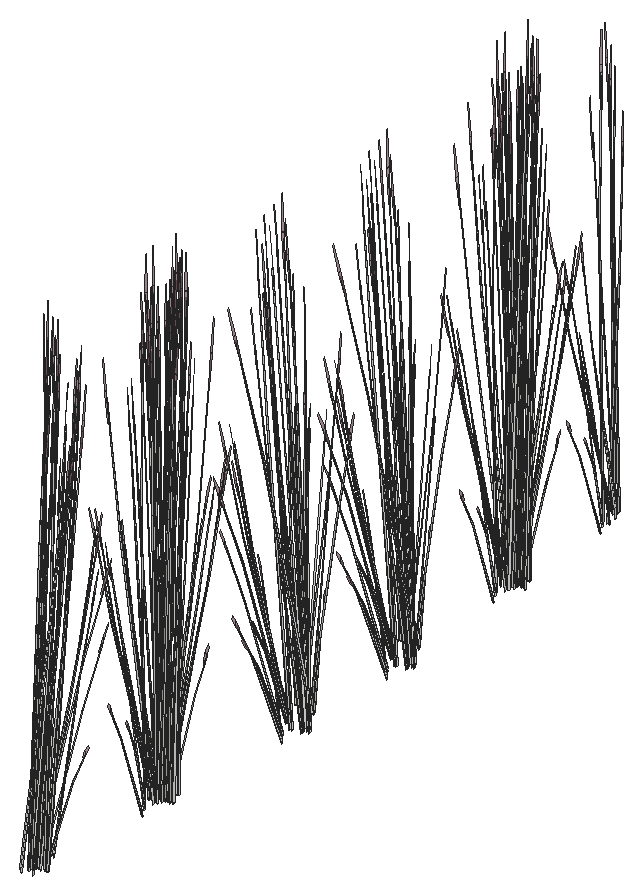
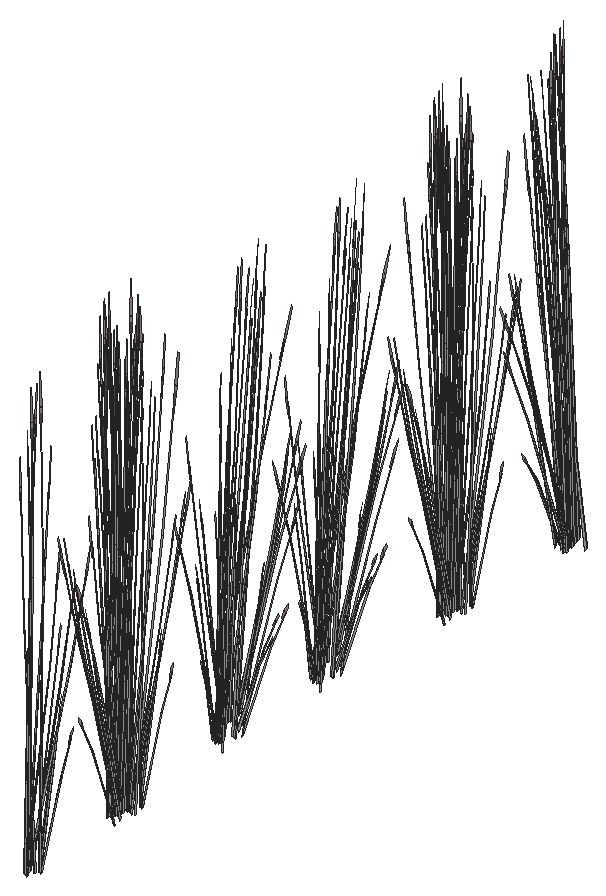
# SketchUp Ruby script. Lengths in inches.
U = 1.inch
M = Sketchup.active_model
def pt(a) = Geom::Point3d.new(a.map { |v| v * U })
def face(e, loops, mat)
  f = e.add_face(loops[0].map { |a| pt(a) })
  loops[1..].each { |l| e.add_face(l.map { |a| pt(a) }).erase! }
  f.material = f.back_material = mat if mat
  f
end
# faces: each face lists its corners as indices into pts; further lists are holes
def faces(e, pts, list, mat = nil) = list.each { |f| face(e, (f[0].is_a?(Array) ? f : [f]).map { |l| l.map { |i| pts[i] } }, mat) }
# xy, xz, yz: faces in a plane at the given z, y or x. An outline is a flat list of corners, or four numbers for a rectangle; further outlines are holes
def ring(l) = l.size == 4 ? [[l[0], l[1]], [l[2], l[1]], [l[2], l[3]], [l[0], l[3]]] : l.each_slice(2).to_a
def flat(e, list, mat, &to3) = list.each { |f| face(e, (f[0].is_a?(Array) ? f : [f]).map { |l| ring(l).map { |u, v| to3.(u, v) } }, mat) }
def xy(e, z, list, mat = nil) = flat(e, list, mat) { |x, y| [x, y, z] }
def xz(e, y, list, mat = nil) = flat(e, list, mat) { |x, z| [x, y, z] }
def yz(e, x, list, mat = nil) = flat(e, list, mat) { |y, z| [x, y, z] }
def lines(e, pts, list) = list.each { |a, b| e.add_line(pt(pts[a]), pt(pts[b])) }
# prism: a flat outline (further loops are holes) pulled along v
def prism(e, loops, v, mat = nil)
  f = face(e, loops, mat); d = Geom::Vector3d.new(v.map { |x| x * U })
  f.pushpull(f.normal.samedirection?(d) ? d.length : -d.length)
end
def box(e, o, s, mat = nil) = prism(e, [[o, [o[0] + s[0], o[1], o[2]], [o[0] + s[0], o[1] + s[1], o[2]], [o[0], o[1] + s[1], o[2]]]], [0, 0, s[2]], mat)
def at(x, y, z, deg = 0) = Geom::Transformation.translation(pt([x, y, z])) * Geom::Transformation.rotation(ORIGIN, Z_AXIS, deg.degrees)
def axes(o, x, y, z) = Geom::Transformation.new([*x, 0, *y, 0, *z, 0, *pt(o).to_a, 1])
def part(name) = M.definitions.add(name)
# library, detail: a bought-in or finely detailed component or shape, given as its bounding box
def library(name, o, s) = part(name).tap { |d| box(d.entities, o, s) }
def detail(e, o, s) = box(e.add_group.entities, o, s)
def put(e, d, t, mat = nil) = e.add_instance(d, t).tap { |i| i.material = mat if mat }
def group(e, t, mat = nil) = e.add_group.tap { |g| g.transformation = t; g.material = mat if mat }.entities
root = M.entities
M.materials.add("LightPink_Translucent").color = [144, 107, 117]
M.materials["LightPink_Translucent"].alpha = 0.75
c1 = part("blade")
p = [[2.15,0.21,22],[0,0.17,0],[0.09,0.45,0],[2.18,0.31,22],[2.29,0.31,22],[0.38,0.45,0],
  [2.48,0.24,33],[2.49,0.24,33],[2.48,0.22,33]]
faces(c1.entities,p,[[0,1,2,3],[4,5,2,3],[6,3,4,7],[8,0,3,6]])
c2 = part("seeds")
p = [[0.3,-0.1,1.38],[-0.01,-0.03,1.59],[-0.01,-0.03,0.03],[0.14,-0.07,-0.07],[0.29,-0.03,3],[0.15,0.01,3.11]]
faces(c2.entities,p,[[0,1,2,3],[1,0,4,5]],"LightPink_Translucent")
c3 = part("blade with seeds")
put(c3.entities,c1,at(0,0,0))
put(c3.entities,c2,axes([2.4,0.25,30.99],[1.5799,-0.05474,1.17369],[-0.12525,1.92788,0.29478],[-0.07173,-0.02425,1.56792]))
put(root,c3,axes([397.25,199,1.59],[-0.3474,0.18671,1.28929],[-0.11057,-0.53572,0.50096],[0.21332,0.00891,1.46642]))
put(root,c3,axes([398.18,199.14,2.62],[0.06809,-0.4162,0.1448],[0.33266,0.07225,-0.41347],[0.06054,0.04274,1.26744]))
put(root,c3,axes([398.04,199.25,2.72],[-0.21202,-0.39143,0.44739],[0.32115,-0.27564,-0.21531],[0.06861,0.04843,1.43643]))
put(root,c3,axes([398.15,199.27,2.67],[0.35635,-0.30962,-0.29095],[0.23697,0.43749,-0.50002],[0.08792,0.04443,1.59708]))
put(root,c3,axes([398.42,199.78,2.21],[0.39487,0,0],[0,0.48281,0],[0,0,1.78407]))
put(root,c3,axes([398.53,198.65,2.47],[-0.37926,0.12378,0.17642],[-0.09365,-0.46065,0.35086],[0.03382,0.06712,1.60407]))
put(root,c3,axes([398.95,198.625,2.03],[0.08291,0.40636,-0.30978],[-0.32928,0.11539,0.30978],[0.06638,0.04686,1.38974]))
put(root,c3,axes([398.29,199.53,2.38],[-0.44609,-0.09826,0.49198],[0.09078,-0.55493,0.19306],[0.06519,0.05359,1.70813]))
put(root,c3,axes([398.37,200.85,2.18],[0.37054,-0.15823,-0.19198],[0.1302,0.45581,0.00008],[0.0409,-0.01749,1.73897]))
put(root,c3,axes([398.41,199.99,2.21],[0.24637,0.30123,0],[-0.24637,0.30123,0],[0,0,1.69266]))
put(root,c3,axes([398.41,199.63,2.72],[0.17124,-0.42022,0.44739],[0.35581,0.20224,-0.21531],[0,0.09687,1.43643]))
put(root,c3,axes([398.34,199.875,2.29],[0,0.53934,-0.05637],[-0.44133,0,0],[0,0.01695,1.79368]))
put(root,c3,axes([398.37,199.49,2.21],[0.21202,0.39143,-0.44739],[-0.32115,0.27564,0.21531],[0.06861,0.04843,1.43643]))
put(root,c3,axes([399.3,199.87,2.48],[0,-0.46636,0.49651],[0.39487,0,0],[0,0.10622,1.57504]))
put(root,c3,axes([398.55,199.73,2.62],[0.32884,-0.136,0.1448],[0.11516,0.38837,-0.41347],[0,0.08547,1.26744]))
put(root,c3,axes([398.26,201.09,2.2],[0.35581,0.20937,0],[-0.17124,0.43505,0],[0,0,1.74954]))
put(root,c3,axes([398.13,200.92,2.29],[0.15345,0.53576,-0.06012],[-0.43845,0.18773,0],[0.00536,0.01871,1.72173]))
put(root,c3,axes([399.57,199.95,2.375],[0.44133,0,0],[0,0.52122,-0.51607],[0,0.11871,1.63711]))
put(root,c3,axes([399.4,200.22,2.2],[-0.44111,-0.00373,-0.04976],[0,-0.52122,0.49943],[-0.01386,0.11865,1.58352]))
put(root,c3,axes([398.44,199.76,2.67],[0.39748,0.22252,-0.29095],[-0.19139,0.46966,-0.50002],[0.01249,0.11531,1.59708]))
put(root,c3,axes([399.3,200.29,2.03],[-0.24637,0.29097,-0.30978],[-0.24637,-0.29097,0.30978],[0,0.09372,1.38974]))
put(root,c3,axes([399.47,200.3,2.02],[0,0.46636,-0.49651],[-0.39487,0,0],[0,0.10622,1.57504]))
put(root,c3,axes([398.97,201.27,2.77],[-0.19872,-0.13409,1.1486],[0.2566,-0.13625,0.84392],[0.06921,0.11541,0.25299]))
put(root,c3,axes([398.6,200.24,2.09],[0.12941,0.42699,-0.69212],[-0.37279,0.15378,-0.18165],[0.0143,0.14459,1.52773]))
put(root,c3,axes([399,201.88,2.67],[-0.22633,-0.01463,1.0506],[0.14947,-0.31064,0.58006],[0.08941,0.11036,0.8241]))
put(root,c3,axes([398.27,201.125,2.59],[0.00623,-0.15459,1.43002],[0.29764,-0.17268,-0.30754],[0.09188,0.18503,0.61141]))
put(root,c3,axes([397.75,201.65,4.68],[0.34695,0.11691,-0.51099],[-0.11892,0.40083,-0.3958],[0.03181,0.16138,0.97773]))
put(root,c3,axes([397.95,200.82,3.875],[-0.08068,-0.14973,1.71376],[0.3728,-0.12606,0.13857],[0.08426,0.23506,0.73262]))
put(root,c3,axes([397.625,201.57,4.98],[0.16845,0.3792,-0.71045],[-0.34676,0.21133,0.08574],[0.03939,0.18322,1.00501]))
put(root,c3,axes([399.53,216.83,4.98],[-0.16845,-0.3792,-0.71045],[0.34676,-0.21133,0.08574],[-0.03939,-0.18322,1.00501]))
put(root,c3,axes([399.24,215.99,1.49],[-0.0592,0.0168,1.76342],[-0.32738,-0.18913,-0.26939],[0.00549,-0.15776,0.30037]))
put(root,c3,axes([399.57,216.51,4.53],[0.1064,-0.35863,-0.35414],[0.31043,0.1046,0.4572],[-0.02846,-0.14439,0.87481]))
put(root,c3,axes([399.41,216.75,4.68],[-0.34695,-0.11691,-0.51099],[0.11892,-0.40083,-0.3958],[-0.03181,-0.16138,0.97773]))
put(root,c3,axes([399.62,215.75,2.77],[0.04528,0.27194,1.1486],[-0.25117,-0.15062,0.84392],[0.02703,-0.13924,0.25299]))
put(root,c3,axes([400.16,217.06,4.68],[-0.25266,-0.31335,-0.51099],[0.2669,-0.27442,-0.3958],[0.03844,-0.15921,0.97773]))
put(root,c3,axes([398.76,218.25,2.1],[-0.14494,-0.47823,-0.69835],[0.41752,-0.17223,-0.18329],[-0.01602,-0.16194,1.54149]))
put(root,c3,axes([398.7,216.88,2.375],[-0.22066,-0.46731,0],[0.36918,-0.26061,-0.51607],[0.08408,-0.05936,1.63711]))
put(root,c3,axes([399.18,216.32,2.13],[-0.2439,0.26754,-0.03893],[-0.22348,-0.29302,-0.17649],[-0.01573,-0.08303,0.58215]))
put(root,c3,axes([398.98,218.38,2.21],[0.17124,-0.42022,-0.44739],[0.35581,0.20224,0.21531],[0,-0.09687,1.43643]))
put(root,c3,axes([399.13,218.17,2.67],[-0.04113,-0.53214,-0.29095],[0.42835,-0.03218,-0.50002],[0.07543,-0.07088,1.59708]))
put(root,c3,axes([398.07,218.2,2.03],[0.24637,-0.29097,-0.30978],[0.24637,0.29097,0.30978],[0,-0.09372,1.38974]))
put(root,c3,axes([399.1875,218.59,2.43],[0.39767,0.22603,0.24065],[-0.19139,0.46966,0.50002],[0,-0.10827,1.60543]))
put(root,c3,axes([399.06,218.27,2.72],[-0.38326,0.02879,0.44739],[-0.03466,-0.47788,-0.21531],[0.06861,-0.04843,1.43643]))
put(root,c3,axes([399.05,218.44,2.36],[0.15345,0.52148,0.45755],[-0.43845,0.18134,0.17955],[0.00536,-0.09582,1.58856]))
put(root,c3,axes([398.97,218.85,2.72],[-0.17124,0.42022,0.44739],[-0.35581,-0.20224,-0.21531],[0,-0.09687,1.43643]))
put(root,c3,axes([399.6,218.49,2.21],[0,-0.53961,0],[0.44133,0,0],[0,0,1.79456]))
put(root,c3,axes([399.39,218.15,2.36],[-0.29264,0.42323,0.45755],[-0.34767,-0.3736,0.17955],[0.07055,-0.04224,1.58856]))
put(root,c3,axes([399.71,218.91,2.3],[-0.32829,-0.4014,-0.06131],[0.32849,-0.40164,0],[-0.01146,-0.01402,1.75571]))
put(root,c3,axes([398.88,217.45,2.47],[-0.10196,0.46348,0.17642],[-0.3731,-0.13116,0.35086],[0.06445,-0.00226,1.60407]))
put(root,c3,axes([399.09,218.95,2.36],[0.44609,0.09826,0.45755],[-0.09078,0.55493,0.17955],[-0.06519,-0.05359,1.58856]))
put(root,c3,axes([399.52,218.08,2.72],[-0.21202,-0.39143,0.44739],[0.32115,-0.27564,-0.21531],[0.06861,0.04843,1.43643]))
put(root,c3,axes([398.85,219.84,2.47],[0.37926,-0.12378,0.17642],[0.09365,0.46065,0.35086],[-0.03382,-0.06712,1.60407]))
put(root,c3,axes([399.9,218.61,2.21],[0.39487,0,0],[0,0.48281,0],[0,0,1.78407]))
put(root,c3,axes([400.01,217.48,2.47],[-0.37926,0.12378,0.17642],[-0.09365,-0.46065,0.35086],[0.03382,0.06712,1.60407]))
put(root,c3,axes([399.77,218.36,2.38],[-0.44609,-0.09826,0.49198],[0.09078,-0.55493,0.19306],[0.06519,0.05359,1.70813]))
put(root,c3,axes([399.42,219.73,2.2],[-0.11516,-0.40207,0],[0.32884,-0.1408,0],[0,0,1.54371]))
put(root,c3,axes([399.97,219.87,2.47],[0.10196,-0.46348,0.17642],[0.3731,0.13116,0.35086],[-0.06445,0.00226,1.60407]))
put(root,c3,axes([399.89,218.82,2.21],[0.24637,0.30123,0],[-0.24637,0.30123,0],[0,0,1.69266]))
put(root,c3,axes([400.56,218.68,2.47],[-0.2773,-0.3397,0.17642],[0.27945,-0.32949,0.35086],[-0.03063,0.06937,1.60407]))
put(root,c3,axes([399.33,219.91,2.2],[-0.35581,-0.20937,0],[0.17124,-0.43505,0],[0,0,1.62707]))
put(root,c3,axes([399.89,218.46,2.72],[0.17124,-0.42022,0.44739],[0.35581,0.20224,-0.21531],[0,0.09687,1.43643]))
put(root,c3,axes([399.82,218.7,2.29],[0,0.53934,-0.05637],[-0.44133,0,0],[0,0.01695,1.79368]))
put(root,c3,axes([399.8,219.05,2.72],[0.38326,-0.02879,0.44739],[0.03466,0.47788,-0.21531],[-0.06861,0.04843,1.43643]))
put(root,c3,axes([400.03,218.56,2.62],[0.32884,-0.136,0.1448],[0.11516,0.38837,-0.41347],[0,0.08547,1.26744]))
put(root,c3,axes([399.74,219.92,2.2],[0.35581,0.20937,0],[-0.17124,0.43505,0],[0,0,1.74954]))
put(root,c3,axes([399.8,219.25,2.62],[0.26075,0.2802,0.1448],[-0.2175,0.31612,-0.41347],[-0.06054,0.04274,1.26744]))
put(root,c3,axes([400.08,220.11,2.48],[0.33032,-0.23318,0.49651],[0.19744,0.41812,0],[-0.07523,0.05311,1.57504]))
put(root,c3,axes([399.61,219.75,2.29],[0.15345,0.53576,-0.06012],[-0.43845,0.18773,0],[0.00536,0.01871,1.72173]))
put(root,c3,axes([400.875,219.04,2.2],[-0.44111,-0.00373,-0.04976],[0,-0.52122,0.49943],[-0.01386,0.11865,1.58352]))
put(root,c3,axes([400.79,219.12,2.03],[-0.24637,0.29097,-0.30978],[-0.24637,-0.29097,0.30978],[0,0.09372,1.38974]))
put(root,c3,axes([399.72,219.15,2.67],[0.04113,0.53214,-0.29095],[-0.42835,0.03218,-0.50002],[-0.07543,0.07088,1.59708]))
put(root,c3,axes([399.88,218.94,2.21],[-0.17124,0.42022,-0.44739],[-0.35581,-0.20224,0.21531],[0,0.09687,1.43643]))
put(root,c3,axes([399.89,220.14,2.33],[0.44186,0.15158,0.30756],[-0.11054,0.54181,-0.36492],[-0.07313,0.06781,1.64885]))
put(root,c3,axes([400.16,220.4375,2.375],[0.22066,0.46731,0],[-0.36918,0.26061,-0.51607],[-0.08408,0.05936,1.63711]))
put(root,c3,axes([400.08,219.07,2.09],[0.12941,0.42699,-0.69212],[-0.37279,0.15378,-0.18165],[0.0143,0.14459,1.52773]))
put(root,c3,axes([399,220.58,1.49],[0.05712,-0.02538,1.76342],[0.34359,0.13968,-0.26939],[0.01005,0.15742,0.30037]))
put(root,c3,axes([398.21,220.64,2.82],[0.32063,-0.08258,0.06507],[0.07371,0.33271,-0.86304],[-0.02033,0.16842,0.7736]))
put(root,c3,axes([399.23,220.48,4.68],[0.34695,0.11691,-0.51099],[-0.11892,0.40083,-0.3958],[0.03181,0.16138,0.97773]))
put(root,c3,axes([399.07,220.72,4.53],[-0.1064,0.35863,-0.35414],[-0.31043,-0.1046,0.4572],[0.02846,0.14439,0.87481]))
put(root,c3,axes([398.77,219.72,3.875],[-0.00864,-0.17899,1.71376],[0.37441,0.11874,0.13857],[-0.02316,0.25508,0.73262]))
put(root,c3,axes([399.1,220.4,4.98],[0.16845,0.3792,-0.71045],[-0.34676,0.21133,0.08574],[0.03939,0.18322,1.00501]))
put(root,c3,axes([401.27,236.43,3.875],[0.08068,0.14973,1.71376],[-0.3728,0.12606,0.13857],[-0.08426,-0.23506,0.73262]))
put(root,c3,axes([401.17,236.04,2.59],[-0.02137,0.15256,1.43002],[-0.31245,0.12771,-0.30754],[-0.07303,-0.19719,0.61141]))
put(root,c3,axes([401.0625,235.79,2.77],[0.18411,0.16231,1.1486],[-0.26813,0.09757,0.84392],[-0.05737,-0.12474,0.25299]))
put(root,c3,axes([401.51,236.65,4.98],[-0.30095,-0.22541,-0.71045],[0.21388,-0.395,0.08574],[-0.10904,-0.13459,1.00501]))
put(root,c3,axes([401.4,236.36,4.53],[-0.05451,-0.37564,-0.35414],[0.31161,-0.09919,0.4572],[-0.0837,-0.10765,0.87481]))
put(root,c3,axes([400.92,236.28,1.49],[-0.03419,0.06144,1.76342],[-0.3455,0.13246,-0.26939],[-0.08346,-0.12049,0.30037]))
put(root,c3,axes([401.37,236.66,4.68],[-0.34827,0.11086,-0.51099],[-0.06092,-0.41983,-0.3958],[-0.09354,-0.12031,0.97773]))
put(root,c3,axes([402.23,239.2,3.33],[0.305,0.18805,1.51261],[-0.29879,0.40513,0.59816],[-0.13384,-0.24012,1.26806]))
put(root,c3,axes([400.68,237.02,4.53],[-0.20082,-0.29199,-0.35414],[0.2293,-0.2764,0.4572],[-0.1165,-0.04206,0.87481]))
put(root,c3,axes([400.7,236.52,2.13],[-0.10181,0.3808,-0.03893],[-0.31336,-0.11714,-0.17649],[-0.04758,-0.06228,0.58215]))
put(root,c3,axes([400.53,238.26,2.375],[-0.44133,0,0],[0,-0.52122,-0.51607],[0,-0.11871,1.63711]))
put(root,c3,axes([400.875,238.12,2.33],[-0.32829,0.39208,0.30756],[-0.32849,-0.38796,-0.36492],[-0.01146,-0.11134,1.64885]))
put(root,c3,axes([400.2,237.72,2.77],[0.22533,-0.03337,1.1486],[-0.14293,0.29403,0.84392],[-0.11135,-0.04411,0.25299]))
put(root,c3,axes([401.73,238.71,2.21],[-0.21202,-0.39143,-0.44739],[0.32115,-0.27564,0.21531],[-0.06861,-0.04843,1.43643]))
put(root,c3,axes([401.54,238.86,2.06],[-0.36714,-0.07646,-0.62353],[0.07747,-0.47163,-0.16365],[-0.10956,-0.05715,1.37633]))
put(root,c3,axes([401.15,239.58,2.03],[-0.08291,-0.40636,-0.30978],[0.32928,-0.11539,0.30978],[-0.06638,-0.04686,1.38974]))
put(root,c3,axes([401.0625,239.76,2.02],[-0.33032,-0.23318,-0.49651],[0.19744,-0.41812,0],[-0.07523,-0.05311,1.57504]))
put(root,c3,axes([401.96,238.93,2.67],[-0.35635,0.30962,-0.29095],[-0.23697,-0.43749,-0.50002],[-0.08792,-0.04443,1.59708]))
put(root,c3,axes([402.36,239.07,2.46],[-0.34464,-0.37536,-0.25192],[0.29,-0.42149,0.5513],[-0.0928,0.04391,1.68216]))
put(root,c3,axes([401.45,239.79,2.48],[0.33032,0.23318,0.49651],[-0.19744,0.41812,0],[-0.07523,-0.05311,1.57504]))
put(root,c3,axes([401.26,240.04,2.375],[-0.22066,0.46731,0],[-0.36918,-0.26061,-0.51607],[-0.08408,-0.05936,1.63711]))
put(root,c3,axes([402.1875,238.99,2.21],[-0.38326,0.02879,-0.44739],[-0.03466,-0.47788,0.21531],[-0.06861,0.04843,1.43643]))
put(root,c3,axes([400.43,239.125,4.53],[-0.30722,0.06665,-0.35414],[-0.08112,-0.381,0.4572],[-0.08804,0.10234,0.87481]))
put(root,c3,axes([402.2,239.27,2.06],[-0.23773,0.35053,-0.62353],[-0.29532,-0.31785,-0.16365],[-0.09526,0.08744,1.37633]))
put(root,c3,axes([400.97,238.75,3.875],[0.08815,-0.14329,1.71376],[0.22258,0.38678,0.13857],[-0.15267,0.17614,0.73262]))
put(root,c3,axes([400.6875,239.17,4.68],[0.09067,0.42583,-0.51099],[-0.34336,0.07449,-0.3958],[-0.0984,0.11438,0.97773]))
put(root,c3,axes([400.27,240.25,1.49],[0.04734,0.04659,1.76342],[0.08027,0.4317,-0.26939],[-0.10492,0.09206,0.30037]))
put(root,c3,axes([400.9,239.1,3.875],[0.06572,-0.16029,1.71376],[0.27569,0.33172,0.13857],[-0.12437,0.20675,0.73262]))
put(root,c3,axes([400.98,240.01,4.53],[-0.23881,0.24554,-0.35414],[-0.22606,-0.28036,0.4572],[-0.0344,0.14245,0.87481]))
put(root,c3,axes([401.13,240.96,2.77],[-0.00913,-0.2773,1.1486],[0.22824,0.19778,0.84392],[-0.04489,0.13217,0.25299]))
put(root,c3,axes([401.13,239.75,5.34],[-0.00918,0.43138,-0.7886],[-0.38672,-0.02897,0.09517],[-0.04081,0.18275,1.11556]))
put(root,c3,axes([400.86,240.71,2.59],[0.11138,-0.07357,1.43002],[0.27499,0.22183,-0.30754],[-0.08185,0.19194,0.61141]))
put(root,c3,axes([401.01,240.35,3.36],[0.00775,-0.24075,1.54345],[0.34877,0.12716,0.21329],[-0.03022,0.25658,0.72882]))
put(root,c3,axes([401.27,253.3125,3.875],[0.08068,0.14973,1.71376],[-0.3728,0.12606,0.13857],[-0.08426,-0.23506,0.73262]))
put(root,c3,axes([401.17,252.92,2.59],[-0.02137,0.15256,1.43002],[-0.31245,0.12771,-0.30754],[-0.07303,-0.19719,0.61141]))
put(root,c3,axes([401.0625,252.67,2.77],[0.18411,0.16231,1.1486],[-0.26813,0.09757,0.84392],[-0.05737,-0.12474,0.25299]))
put(root,c3,axes([401.51,253.53,4.98],[-0.30095,-0.22541,-0.71045],[0.21388,-0.395,0.08574],[-0.10904,-0.13459,1.00501]))
put(root,c3,axes([401.4,253.23,4.53],[-0.05451,-0.37564,-0.35414],[0.31161,-0.09919,0.4572],[-0.0837,-0.10765,0.87481]))
put(root,c3,axes([400.92,253.16,1.49],[-0.03419,0.06144,1.76342],[-0.3455,0.13246,-0.26939],[-0.08346,-0.12049,0.30037]))
put(root,c3,axes([401.37,253.54,4.68],[-0.34827,0.11086,-0.51099],[-0.06092,-0.41983,-0.3958],[-0.09354,-0.12031,0.97773]))
put(root,c3,axes([402.23,256.08,3.33],[0.305,0.18805,1.51261],[-0.29879,0.40513,0.59816],[-0.13384,-0.24012,1.26806]))
put(root,c3,axes([400.68,253.89,4.53],[-0.20082,-0.29199,-0.35414],[0.2293,-0.2764,0.4572],[-0.1165,-0.04206,0.87481]))
put(root,c3,axes([400.7,253.4,2.13],[-0.10181,0.3808,-0.03893],[-0.31336,-0.11714,-0.17649],[-0.04758,-0.06228,0.58215]))
put(root,c3,axes([400.53,255.14,2.375],[-0.44133,0,0],[0,-0.52122,-0.51607],[0,-0.11871,1.63711]))
put(root,c3,axes([400.875,255,2.33],[-0.32829,0.39208,0.30756],[-0.32849,-0.38796,-0.36492],[-0.01146,-0.11134,1.64885]))
put(root,c3,axes([400.2,254.59,2.77],[0.22533,-0.03337,1.1486],[-0.14293,0.29403,0.84392],[-0.11135,-0.04411,0.25299]))
put(root,c3,axes([401.73,255.59,2.21],[-0.21202,-0.39143,-0.44739],[0.32115,-0.27564,0.21531],[-0.06861,-0.04843,1.43643]))
put(root,c3,axes([401.54,255.74,2.06],[-0.36714,-0.07646,-0.62353],[0.07747,-0.47163,-0.16365],[-0.10956,-0.05715,1.37633]))
put(root,c3,axes([401.15,256.46,2.03],[-0.08291,-0.40636,-0.30978],[0.32928,-0.11539,0.30978],[-0.06638,-0.04686,1.38974]))
put(root,c3,axes([401.0625,256.63,2.02],[-0.33032,-0.23318,-0.49651],[0.19744,-0.41812,0],[-0.07523,-0.05311,1.57504]))
put(root,c3,axes([401.96,255.8125,2.67],[-0.35635,0.30962,-0.29095],[-0.23697,-0.43749,-0.50002],[-0.08792,-0.04443,1.59708]))
put(root,c3,axes([402.36,255.95,2.46],[-0.34464,-0.37536,-0.25192],[0.29,-0.42149,0.5513],[-0.0928,0.04391,1.68216]))
put(root,c3,axes([401.45,256.67,2.48],[0.33032,0.23318,0.49651],[-0.19744,0.41812,0],[-0.07523,-0.05311,1.57504]))
put(root,c3,axes([401.26,256.92,2.375],[-0.22066,0.46731,0],[-0.36918,-0.26061,-0.51607],[-0.08408,-0.05936,1.63711]))
put(root,c3,axes([402.1875,255.87,2.21],[-0.38326,0.02879,-0.44739],[-0.03466,-0.47788,0.21531],[-0.06861,0.04843,1.43643]))
put(root,c3,axes([400.43,256,4.53],[-0.30722,0.06665,-0.35414],[-0.08112,-0.381,0.4572],[-0.08804,0.10234,0.87481]))
put(root,c3,axes([402.2,256.15,2.06],[-0.23773,0.35053,-0.62353],[-0.29532,-0.31785,-0.16365],[-0.09526,0.08744,1.37633]))
put(root,c3,axes([400.97,255.63,3.875],[0.08815,-0.14329,1.71376],[0.22258,0.38678,0.13857],[-0.15267,0.17614,0.73262]))
put(root,c3,axes([400.6875,256.05,4.68],[0.09067,0.42583,-0.51099],[-0.34336,0.07449,-0.3958],[-0.0984,0.11438,0.97773]))
put(root,c3,axes([400.27,257.13,1.49],[0.04734,0.04659,1.76342],[0.08027,0.4317,-0.26939],[-0.10492,0.09206,0.30037]))
put(root,c3,axes([400.9,255.98,3.875],[0.06572,-0.16029,1.71376],[0.27569,0.33172,0.13857],[-0.12437,0.20675,0.73262]))
put(root,c3,axes([400.98,256.88,4.53],[-0.23881,0.24554,-0.35414],[-0.22606,-0.28036,0.4572],[-0.0344,0.14245,0.87481]))
put(root,c3,axes([401.13,257.84,2.77],[-0.00913,-0.2773,1.1486],[0.22824,0.19778,0.84392],[-0.04489,0.13217,0.25299]))
put(root,c3,axes([401.13,256.625,5.34],[-0.00918,0.43138,-0.7886],[-0.38672,-0.02897,0.09517],[-0.04081,0.18275,1.11556]))
put(root,c3,axes([400.86,257.59,2.59],[0.11138,-0.07357,1.43002],[0.27499,0.22183,-0.30754],[-0.08185,0.19194,0.61141]))
put(root,c3,axes([401.01,257.23,3.36],[0.00775,-0.24075,1.54345],[0.34877,0.12716,0.21329],[-0.03022,0.25658,0.72882]))
put(root,c3,axes([399.74,273.125,4.98],[-0.16845,-0.3792,-0.71045],[0.34676,-0.21133,0.08574],[-0.03939,-0.18322,1.00501]))
put(root,c3,axes([399.45,272.29,1.49],[-0.0592,0.0168,1.76342],[-0.32738,-0.18913,-0.26939],[0.00549,-0.15776,0.30037]))
put(root,c3,axes([399.78,272.8,4.53],[0.1064,-0.35863,-0.35414],[0.31043,0.1046,0.4572],[-0.02846,-0.14439,0.87481]))
put(root,c3,axes([399.62,273.05,4.68],[-0.34695,-0.11691,-0.51099],[0.11892,-0.40083,-0.3958],[-0.03181,-0.16138,0.97773]))
put(root,c3,axes([399.83,272.05,2.77],[0.04528,0.27194,1.1486],[-0.25117,-0.15062,0.84392],[0.02703,-0.13924,0.25299]))
put(root,c3,axes([398.97,274.55,2.1],[-0.14494,-0.47823,-0.69835],[0.41752,-0.17223,-0.18329],[-0.01602,-0.16194,1.54149]))
put(root,c3,axes([398.91,273.18,2.375],[-0.22066,-0.46731,0],[0.36918,-0.26061,-0.51607],[0.08408,-0.05936,1.63711]))
put(root,c3,axes([399.39,272.61,2.13],[-0.2439,0.26754,-0.03893],[-0.22348,-0.29302,-0.17649],[-0.01573,-0.08303,0.58215]))
put(root,c3,axes([399.1875,274.67,2.21],[0.17124,-0.42022,-0.44739],[0.35581,0.20224,0.21531],[0,-0.09687,1.43643]))
put(root,c3,axes([398.28,274.49,2.03],[0.24637,-0.29097,-0.30978],[0.24637,0.29097,0.30978],[0,-0.09372,1.38974]))
put(root,c3,axes([399.14,275.02,2.67],[-0.39748,-0.22252,-0.29095],[0.19139,-0.46966,-0.50002],[-0.01249,-0.11531,1.59708]))
put(root,c3,axes([399.4,274.88,2.43],[0.39767,0.22603,0.24065],[-0.19139,0.46966,0.50002],[0,-0.10827,1.60543]))
put(root,c3,axes([399.27,274.57,2.72],[-0.38326,0.02879,0.44739],[-0.03466,-0.47788,-0.21531],[0.06861,-0.04843,1.43643]))
put(root,c3,axes([399.26,274.74,2.36],[0.15345,0.52148,0.45755],[-0.43845,0.18134,0.17955],[0.00536,-0.09582,1.58856]))
put(root,c3,axes([399.18,275.15,2.72],[-0.17124,0.42022,0.44739],[-0.35581,-0.20224,-0.21531],[0,-0.09687,1.43643]))
put(root,c3,axes([399.81,274.78,2.21],[0,-0.53961,0],[0.44133,0,0],[0,0,1.79456]))
put(root,c3,axes([399.6,274.44,2.36],[-0.29264,0.42323,0.45755],[-0.34767,-0.3736,0.17955],[0.07055,-0.04224,1.58856]))
put(root,c3,axes([399.92,275.2,2.3],[-0.32829,-0.4014,-0.06131],[0.32849,-0.40164,0],[-0.01146,-0.01402,1.75571]))
put(root,c3,axes([399.09,273.75,2.47],[-0.10196,0.46348,0.17642],[-0.3731,-0.13116,0.35086],[0.06445,-0.00226,1.60407]))
put(root,c3,axes([399.29,275.25,2.36],[0.44609,0.09826,0.45755],[-0.09078,0.55493,0.17955],[-0.06519,-0.05359,1.58856]))
put(root,c3,axes([399.06,276.14,2.47],[0.37926,-0.12378,0.17642],[0.09365,0.46065,0.35086],[-0.03382,-0.06712,1.60407]))
put(root,c3,axes([400.22,273.77,2.47],[-0.37926,0.12378,0.17642],[-0.09365,-0.46065,0.35086],[0.03382,0.06712,1.60407]))
put(root,c3,axes([399.98,274.66,2.38],[-0.44609,-0.09826,0.49198],[0.09078,-0.55493,0.19306],[0.06519,0.05359,1.70813]))
put(root,c3,axes([399.625,276.03,2.2],[-0.11516,-0.40207,0],[0.32884,-0.1408,0],[0,0,1.54371]))
put(root,c3,axes([400.18,276.16,2.47],[0.10196,-0.46348,0.17642],[0.3731,0.13116,0.35086],[-0.06445,0.00226,1.60407]))
put(root,c3,axes([400.1,275.11,2.21],[0.24637,0.30123,0],[-0.24637,0.30123,0],[0,0,1.69266]))
put(root,c3,axes([400.77,274.98,2.47],[-0.2773,-0.3397,0.17642],[0.27945,-0.32949,0.35086],[-0.03063,0.06937,1.60407]))
put(root,c3,axes([399.54,276.21,2.2],[-0.35581,-0.20937,0],[0.17124,-0.43505,0],[0,0,1.62707]))
put(root,c3,axes([400.1,274.76,2.72],[0.17124,-0.42022,0.44739],[0.35581,0.20224,-0.21531],[0,0.09687,1.43643]))
put(root,c3,axes([400.03,275,2.29],[0,0.53934,-0.05637],[-0.44133,0,0],[0,0.01695,1.79368]))
put(root,c3,axes([400.01,275.34,2.72],[0.38326,-0.02879,0.44739],[0.03466,0.47788,-0.21531],[-0.06861,0.04843,1.43643]))
put(root,c3,axes([399.95,276.22,2.2],[0.35581,0.20937,0],[-0.17124,0.43505,0],[0,0,1.74954]))
put(root,c3,axes([400.01,275.55,2.62],[0.26075,0.2802,0.1448],[-0.2175,0.31612,-0.41347],[-0.06054,0.04274,1.26744]))
put(root,c3,axes([400.29,276.41,2.48],[0.33032,-0.23318,0.49651],[0.19744,0.41812,0],[-0.07523,0.05311,1.57504]))
put(root,c3,axes([399.82,276.04,2.29],[0.15345,0.53576,-0.06012],[-0.43845,0.18773,0],[0.00536,0.01871,1.72173]))
put(root,c3,axes([399.99,276.62,2.03],[-0.32928,-0.11539,-0.30978],[0.08291,-0.40636,0.30978],[-0.06638,0.04686,1.38974]))
put(root,c3,axes([401.09,275.34,2.2],[-0.44111,-0.00373,-0.04976],[0,-0.52122,0.49943],[-0.01386,0.11865,1.58352]))
put(root,c3,axes([400.99,275.42,2.03],[-0.24637,0.29097,-0.30978],[-0.24637,-0.29097,0.30978],[0,0.09372,1.38974]))
put(root,c3,axes([399.93,275.44,2.67],[0.04113,0.53214,-0.29095],[-0.42835,0.03218,-0.50002],[-0.07543,0.07088,1.59708]))
put(root,c3,axes([400.09,275.24,2.21],[-0.17124,0.42022,-0.44739],[-0.35581,-0.20224,0.21531],[0,0.09687,1.43643]))
put(root,c3,axes([400.1,276.44,2.33],[0.44186,0.15158,0.30756],[-0.11054,0.54181,-0.36492],[-0.07313,0.06781,1.64885]))
put(root,c3,axes([400.37,276.74,2.375],[0.22066,0.46731,0],[-0.36918,0.26061,-0.51607],[-0.08408,0.05936,1.63711]))
put(root,c3,axes([400.18,274.89,2.84],[-0.00964,-0.43909,1.41272],[0.43635,0.11382,0.59816],[-0.1032,0.24027,1.3335]))
put(root,c3,axes([399.21,276.88,1.49],[0.05712,-0.02538,1.76342],[0.34359,0.13968,-0.26939],[0.01005,0.15742,0.30037]))
put(root,c3,axes([398.69,276.47,5],[0.25266,0.31335,-0.5672],[-0.2669,0.27442,-0.43934],[-0.03844,0.15921,1.08528]))
put(root,c3,axes([398.42,276.94,2.82],[0.32063,-0.08258,0.06507],[0.07371,0.33271,-0.86304],[-0.02033,0.16842,0.7736]))
put(root,c3,axes([399.44,276.77,4.68],[0.34695,0.11691,-0.51099],[-0.11892,0.40083,-0.3958],[0.03181,0.16138,0.97773]))
put(root,c3,axes([399.28,277.02,4.53],[-0.1064,0.35863,-0.35414],[-0.31043,-0.1046,0.4572],[0.02846,0.14439,0.87481]))
put(root,c3,axes([398.98,276.02,3.875],[-0.00864,-0.17899,1.71376],[0.37441,0.11874,0.13857],[-0.02316,0.25508,0.73262]))
put(root,c3,axes([399.3125,276.7,4.98],[0.16845,0.3792,-0.71045],[-0.34676,0.21133,0.08574],[0.03939,0.18322,1.00501]))
put(root,c3,axes([399.76,290.5625,2.59],[-0.10032,0.0944,1.43002],[-0.30046,-0.16522,-0.30754],[0.05569,-0.20547,0.61141]))
put(root,c3,axes([399.3,290.89,4.98],[-0.16845,-0.3792,-0.71045],[0.34676,-0.21133,0.08574],[-0.03939,-0.18322,1.00501]))
put(root,c3,axes([399.01,290.05,1.49],[-0.0592,0.0168,1.76342],[-0.32738,-0.18913,-0.26939],[0.00549,-0.15776,0.30037]))
put(root,c3,axes([399.33,290.57,4.53],[0.1064,-0.35863,-0.35414],[0.31043,0.1046,0.4572],[-0.02846,-0.14439,0.87481]))
put(root,c3,axes([399.39,289.81,2.77],[0.04528,0.27194,1.1486],[-0.25117,-0.15062,0.84392],[0.02703,-0.13924,0.25299]))
put(root,c3,axes([399.92,291.12,4.68],[-0.25266,-0.31335,-0.51099],[0.2669,-0.27442,-0.3958],[0.03844,-0.15921,0.97773]))
put(root,c3,axes([398.46,290.94,2.375],[-0.22066,-0.46731,0],[0.36918,-0.26061,-0.51607],[0.08408,-0.05936,1.63711]))
put(root,c3,axes([398.95,290.375,2.13],[-0.2439,0.26754,-0.03893],[-0.22348,-0.29302,-0.17649],[-0.01573,-0.08303,0.58215]))
put(root,c3,axes([398.74,292.4375,2.21],[0.17124,-0.42022,-0.44739],[0.35581,0.20224,0.21531],[0,-0.09687,1.43643]))
put(root,c3,axes([398.9,292.23,2.67],[-0.04113,-0.53214,-0.29095],[0.42835,-0.03218,-0.50002],[0.07543,-0.07088,1.59708]))
put(root,c3,axes([398.84,291.05,2.03],[0.32928,0.11539,-0.30978],[-0.08291,0.40636,0.30978],[0.06638,-0.04686,1.38974]))
put(root,c3,axes([398.95,292.65,2.43],[0.39767,0.22603,0.24065],[-0.19139,0.46966,0.50002],[0,-0.10827,1.60543]))
put(root,c3,axes([398.82,292.33,2.72],[-0.38326,0.02879,0.44739],[-0.03466,-0.47788,-0.21531],[0.06861,-0.04843,1.43643]))
